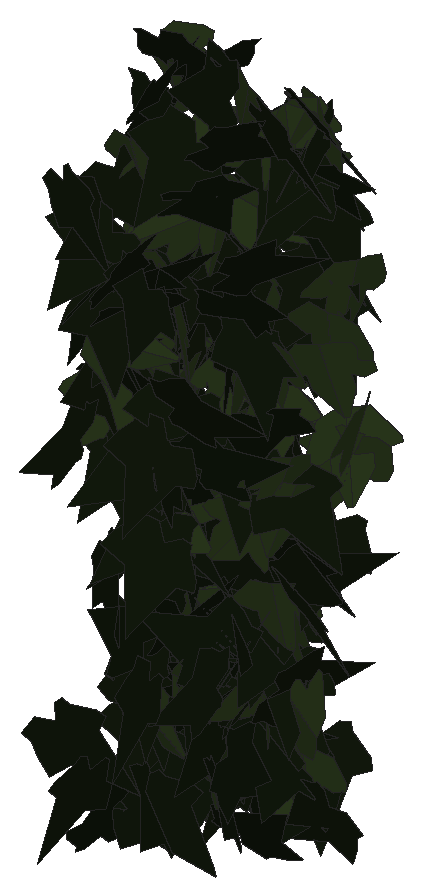
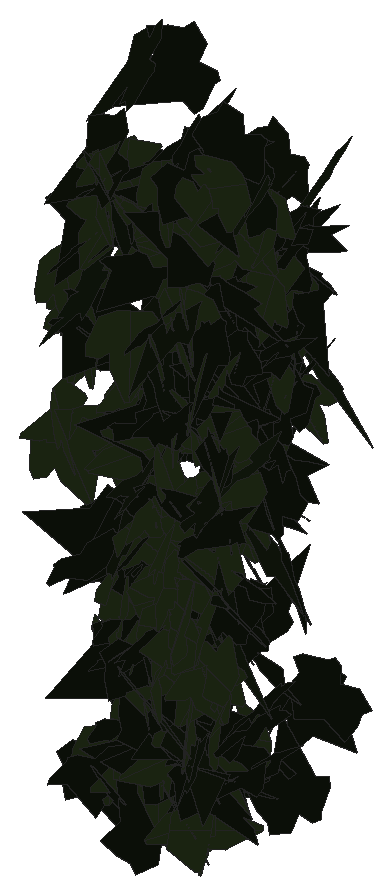
# SketchUp Ruby script. Lengths in inches.
U = 1.inch
M = Sketchup.active_model
def pt(a) = Geom::Point3d.new(a.map { |v| v * U })
def face(e, loops, mat)
  f = e.add_face(loops[0].map { |a| pt(a) })
  loops[1..].each { |l| e.add_face(l.map { |a| pt(a) }).erase! }
  f.material = f.back_material = mat if mat
  f
end
# faces: each face lists its corners as indices into pts; further lists are holes
def faces(e, pts, list, mat = nil) = list.each { |f| face(e, (f[0].is_a?(Array) ? f : [f]).map { |l| l.map { |i| pts[i] } }, mat) }
# xy, xz, yz: faces in a plane at the given z, y or x. An outline is a flat list of corners, or four numbers for a rectangle; further outlines are holes
def ring(l) = l.size == 4 ? [[l[0], l[1]], [l[2], l[1]], [l[2], l[3]], [l[0], l[3]]] : l.each_slice(2).to_a
def flat(e, list, mat, &to3) = list.each { |f| face(e, (f[0].is_a?(Array) ? f : [f]).map { |l| ring(l).map { |u, v| to3.(u, v) } }, mat) }
def xy(e, z, list, mat = nil) = flat(e, list, mat) { |x, y| [x, y, z] }
def xz(e, y, list, mat = nil) = flat(e, list, mat) { |x, z| [x, y, z] }
def yz(e, x, list, mat = nil) = flat(e, list, mat) { |y, z| [x, y, z] }
def lines(e, pts, list) = list.each { |a, b| e.add_line(pt(pts[a]), pt(pts[b])) }
# prism: a flat outline (further loops are holes) pulled along v
def prism(e, loops, v, mat = nil)
  f = face(e, loops, mat); d = Geom::Vector3d.new(v.map { |x| x * U })
  f.pushpull(f.normal.samedirection?(d) ? d.length : -d.length)
end
def box(e, o, s, mat = nil) = prism(e, [[o, [o[0] + s[0], o[1], o[2]], [o[0] + s[0], o[1] + s[1], o[2]], [o[0], o[1] + s[1], o[2]]]], [0, 0, s[2]], mat)
def at(x, y, z, deg = 0) = Geom::Transformation.translation(pt([x, y, z])) * Geom::Transformation.rotation(ORIGIN, Z_AXIS, deg.degrees)
def axes(o, x, y, z) = Geom::Transformation.new([*x, 0, *y, 0, *z, 0, *pt(o).to_a, 1])
def part(name) = M.definitions.add(name)
# library, detail: a bought-in or finely detailed component or shape, given as its bounding box
def library(name, o, s) = part(name).tap { |d| box(d.entities, o, s) }
def detail(e, o, s) = box(e.add_group.entities, o, s)
def put(e, d, t, mat = nil) = e.add_instance(d, t).tap { |i| i.material = mat if mat }
def group(e, t, mat = nil) = e.add_group.tap { |g| g.transformation = t; g.material = mat if mat }.entities
root = M.entities
M.materials.add("efeu1").color = [18, 25, 13]
M.materials.add("efeu2").color = [43, 57, 29]
c1 = part("ivyleaf_9")
p = [[1.54,2.16,1.25],[1.36,2.04,1.19],[-0.21,0.99,0.68],[-0.71,1.11,0.82],[-0.85,0.86,0.67],[-0.8,0.17,0.21],
  [-0.9,-0.01,0.1],[-0.67,-0.16,-0.02],[-0.08,-0.08,-0.05],[-0.03,-0.6,-0.4],[0.65,-0.88,-0.66],[0.83,-0.6,-0.49],
  [1.29,-0.42,-0.43],[1.8125,-0.07,-0.26],[1.21,0.44,0.15]]
faces(c1.entities,p,[[0,1,2,3,4,5,6,7,8,9,10,11,12,13,14]],"efeu1")
c2 = part("ivyleaf_10")
p = [[0,0.5,-0.03],[-0.0625,2.02,-0.43],[-0.19,2.01,-0.46],[-0.54,1.05,-0.29],[-0.52,0.625,-0.18],[-0.83,0.76,-0.28],
  [-1.16,0.64,-0.33],[-1.15,0.33,-0.24],[-0.77,-0.39,0.02],[-0.3,-0.51,0.16],[0.04,-0.48,0.23],[-0.02,2.01,-0.4375],
  [-0.06,2.01,-0.43],[0.04,-0.49,0.23],[0.67,-0.49,0.14],[1.38,0.36,-0.2],[1.375,0.51,-0.24],[0.81,0.65,-0.19],
  [0.62,0.59,-0.15],[0.6,1.09,-0.28],[0.5,1.23,-0.31]]
faces(c2.entities,p,[[0,1,2,3,4,5,6,7,8,9,10],[11,12,0,13,14,15,16,17,18,19,20]],"efeu2")
put(root,c1,axes([7.01,222.2,232.59],[-0.0861,0.39722,-0.16472],[-0.12182,0.13587,0.41345],[0.44549,0.11392,0.08122]))
put(root,c1,axes([6.7,222.25,227.66],[0.03553,-0.01472,0.45084],[0.36359,-0.27327,-0.03622],[0.29539,0.33813,-0.00964]))
put(root,c1,axes([7.11,222.03,228.04],[-0.32073,-0.31158,0.06535],[-0.03827,-0.05301,-0.44751],[0.34115,-0.29888,0.01124]))
put(root,c1,axes([6.91,222.69,224.36],[0.0032,-0.43244,-0.04889],[-0.00048,0.04701,-0.44975],[0.46979,0.00299,-0.00012]))
put(root,c1,axes([7.0625,223.45,227.76],[-0.18053,-0.37603,0.14665],[-0.05909,-0.12998,-0.42796],[0.42968,-0.17587,0.00276]))
put(root,c1,axes([6.99,222.54,223.62],[-0.14612,-0.39297,0.13356],[0.0204,-0.14086,-0.42757],[0.44603,-0.12229,0.06331]))
put(root,c1,axes([6.82,222.83,232.54],[0.18169,-0.38646,0.11189],[0.06107,-0.09265,-0.43809],[0.42892,0.17689,0.01498]))
put(root,c2,axes([7.1,223.21,226.51],[-0.18859,0.36961,0.15468],[-0.06703,0.13518,-0.42513],[-0.42504,-0.18531,-0.00159]))
put(root,c1,axes([7.1,222.16,229.875],[-0.22078,-0.35941,0.14054],[-0.05471,-0.12651,-0.42963],[0.41107,-0.20987,0.0183]))
put(root,c1,axes([7.45,222.82,229.3125],[-0.12494,0.12692,0.41565],[-0.38106,0.19459,-0.17048],[-0.24474,-0.36776,0.05325]))
put(root,c1,axes([6.84,221.78,226.36],[-0.08829,-0.08514,-0.43543],[0.46005,-0.04918,-0.0761],[-0.03566,-0.42374,0.09632]))
put(root,c1,axes([6.8125,220.86,224.3],[-0.02656,-0.02098,-0.45115],[0.31827,0.31835,-0.03339],[0.34454,-0.2957,-0.00394]))
put(root,c1,axes([7.1,221.54,231.39],[-0.08179,-0.2223,0.38081],[-0.13532,-0.34408,-0.2442],[0.44239,-0.14635,-0.00429]))
put(root,c2,axes([7.2,223.46,232.61],[-0.20216,-0.2018,-0.35032],[-0.15461,-0.31241,0.27738],[-0.39489,0.22562,0.07074]))
put(root,c1,axes([7.33,221.87,226.84],[-0.3534,0.27782,-0.0733],[0.05803,-0.04561,-0.44642],[-0.30406,-0.3316,-0.00001]))
put(root,c2,axes([6.8,223.39,225.49],[-0.17295,-0.02757,0.41965],[0.43654,0.00431,0.16714],[-0.01532,0.4341,0.02499]))
put(root,c1,axes([6.98,222.47,224.53],[0.01298,-0.42928,0.07202],[-0.01082,-0.06953,-0.44646],[0.4695,0.01027,-0.01228]))
put(root,c1,axes([7.07,222.28,228.86],[-0.10618,0.02563,0.43989],[-0.04943,-0.43231,0.01618],[0.45497,-0.04099,0.10442]))
put(root,c2,axes([7.16,222,232.21],[-0.46772,0.03923,-0.01202],[0.01235,-0.00189,-0.45224],[-0.0424,-0.43322,0.00088]))
put(root,c2,axes([7.26,221.2,229.75],[-0.26529,0.29838,0.20763],[-0.18922,0.11151,-0.39751],[-0.33842,-0.29625,0.05949]))
put(root,c2,axes([7.2,221.3,229.04],[0.43956,0.01533,-0.1589],[-0.16486,-0.00662,-0.42358],[-0.01801,0.43468,-0.00085]))
put(root,c2,axes([7.4,222.88,228.48],[-0.03279,0.12694,0.43155],[-0.38872,0.22499,-0.09897],[-0.26179,-0.34998,0.09291]))
put(root,c1,axes([7.27,221.23,230.55],[-0.10332,0.35928,-0.23484],[0.07647,-0.21472,-0.38649],[-0.45187,-0.11849,-0.01171]))
put(root,c1,axes([7.02,221.47,222.54],[0.25576,0.28595,0.23572],[-0.15701,-0.17389,0.38613],[0.36145,-0.27788,0.00093]))
put(root,c2,axes([7.18,221.93,230.82],[-0.44666,0.13446,-0.01027],[0.01193,0.00205,-0.45225],[-0.14512,-0.41369,-0.00558]))
put(root,c1,axes([7.01,221.79,231.97],[0.06022,-0.27008,-0.34987],[-0.02363,0.337,-0.28515],[0.46533,0.05206,0.03079]))
put(root,c2,axes([7.16,223.29,225.375],[0.30448,0.30754,-0.12804],[-0.09164,-0.08924,-0.4339],[-0.34584,0.29441,0.00224]))
put(root,c1,axes([7,221.58,229.33],[0.33209,0.24469,0.19401],[0.15576,0.11835,-0.40868],[-0.29354,0.33962,0.00263]))
put(root,c1,axes([7.48,221.77,224.82],[-0.41542,0.05328,-0.20389],[-0.20887,0.03249,0.40382],[0.06718,0.4305,-0.00524]))
put(root,c2,axes([7.45,223.32,222.92],[0.03944,0.06073,-0.49473],[-0.41349,-0.27314,-0.06649],[-0.27834,0.41437,0.02868]))
put(root,c2,axes([6.875,223.14,233.12],[-0.19368,0.00219,-0.41216],[0.42798,-0.00512,-0.18652],[-0.00601,-0.43496,0.00012]))
put(root,c1,axes([6.93,222.91,228.41],[0.0057,-0.43914,0.239],[0.18695,-0.21981,-0.40833],[0.4637,0.09402,0.16169]))
put(root,c1,axes([7.24,223.38,227.88],[0.217,-0.37827,0.079],[-0.03153,0.07049,0.44539],[-0.41549,-0.20291,0.00746]))
put(root,c1,axes([7.12,221.57,229.04],[0.19452,-0.28428,-0.28665],[0.15821,-0.23348,0.34999],[-0.39729,-0.23217,-0.00097]))
put(root,c1,axes([7.45,222.55,225.64],[-0.3255,0.31364,0.00457],[-0.0036,0.0029,-0.45238],[-0.33874,-0.30141,0.00041]))
put(root,c1,axes([7.26,221.32,231.35],[-0.30896,-0.30466,0.12552],[-0.03057,-0.13664,-0.42849],[0.35259,-0.27881,0.07284]))
put(root,c2,axes([7.27,222.34,231.84],[0.21821,0.30996,-0.23791],[-0.15757,-0.1775,-0.38414],[-0.38506,0.24828,0.02238]))
put(root,c2,axes([7.3,223.26,230.14],[-0.28074,0.30803,0.17017],[-0.12216,0.11859,-0.41907],[-0.35633,-0.28334,0.00959]))
put(root,c1,axes([7.5,220.38,228.87],[-0.34524,0.28997,0.05653],[-0.04568,0.03427,-0.44884],[-0.31533,-0.32244,0.00313]))
put(root,c1,axes([7.35,222.44,226.51],[0.01971,0.17276,0.41476],[0.01942,0.39851,-0.1804],[-0.46898,0.02376,0.00996]))
put(root,c1,axes([7.12,222.58,233.54],[0.44489,0.11923,-0.07587],[-0.07445,-0.02421,-0.44597],[-0.13132,0.41764,-0.0042]))
put(root,c1,axes([7.04,220.71,232.24],[0.28743,-0.33046,-0.09969],[-0.06297,0.07612,-0.44127],[0.36624,0.27244,0.00237]))
put(root,c1,axes([6.85,221.91,228.97],[0.2343,-0.16249,0.35384],[0.3202,-0.16898,-0.28055],[0.25157,0.36642,0.02753]))
put(root,c2,axes([7.2,222.625,229.98],[-0.09056,0.42418,-0.0495],[0.00675,-0.04728,-0.44967],[-0.46094,-0.08403,0.00314]))
put(root,c1,axes([7.125,222.78,228.55],[0.1144,0.34859,0.24718],[-0.09401,-0.22172,0.37855],[0.44586,-0.13619,0.0164]))
put(root,c1,axes([7.55,223.03,226.71],[-0.43011,0.15738,0.07959],[-0.07961,0.02168,-0.44529],[-0.17141,-0.40495,0.0071]))
put(root,c1,axes([7.43,223,223.74],[-0.10007,0.30049,-0.3126],[0.01008,-0.30612,-0.32127],[-0.45891,-0.07225,0.06111]))
put(root,c1,axes([6.96,222.11,228.7],[-0.04751,-0.03905,-0.44824],[0.46005,0.07258,-0.05205],[0.08252,-0.42712,0.03213]))
put(root,c1,axes([7.11,222.59,223.98],[0.40028,0.22007,0.06087],[0.06004,0.02099,-0.44816],[-0.23849,0.37464,-0.01065]))
put(root,c2,axes([7,222.7,228.3],[-0.18205,-0.05521,-0.41308],[0.41661,0.09541,-0.18405],[0.11835,-0.4208,0.01247]))
put(root,c1,axes([7.32,223.03,230.66],[0.36273,0.00889,-0.28735],[-0.29807,-0.01401,-0.34938],[-0.01702,0.43468,-0.00538]))
put(root,c1,axes([7.48,223.31,233.16],[-0.11581,0.33752,-0.2627],[-0.01717,-0.26369,-0.35943],[-0.45498,-0.07596,0.08043]))
put(root,c1,axes([7.09,221.73,230.03],[0.13846,0.411,-0.06466],[0.00846,0.06266,0.44761],[0.44885,-0.12797,0.01151]))
put(root,c1,axes([7.38,222.66,230.24],[0.30947,0.20995,-0.26112],[-0.24035,-0.1197,-0.36824],[-0.25918,0.36169,0.0297]))
put(root,c1,axes([7.07,222.88,229.81],[-0.17981,-0.09387,-0.40639],[0.39385,0.14245,-0.19718],[0.18238,-0.40015,0.02514]))
put(root,c1,axes([7.26,222.05,228.01],[-0.29092,0.09172,-0.34218],[0.33517,-0.10928,-0.29593],[-0.15406,-0.41094,0.00233]))
put(root,c1,axes([7.53,222.6,231.04],[-0.46728,-0.02463,0.03915],[-0.04018,-0.00864,-0.45065],[0.02731,-0.43422,0.00674]))
put(root,c2,axes([7,222.85,229.13],[0.21355,0.11427,0.38504],[0.3392,0.19614,-0.23741],[-0.24505,0.37108,0.00691]))
put(root,c2,axes([7.48,222.95,223.62],[0.35413,0.09351,-0.28093],[-0.28817,-0.04734,-0.35389],[-0.11075,0.42219,0.02254]))
put(root,c1,axes([7.2,222.88,225.96],[0.45213,-0.05395,0.10934],[-0.11209,0.01716,0.43897],[-0.06101,-0.4313,0.00379]))
put(root,c2,axes([7.04,222.31,224.01],[-0.14654,0.09861,-0.41742],[0.36626,-0.21489,-0.17414],[-0.25513,-0.36514,-0.01025]))
put(root,c2,axes([7.41,221.57,228.47],[-0.2646,0.34109,0.11792],[-0.10009,0.07264,-0.43551],[-0.37507,-0.26001,0.03302]))
put(root,c1,axes([7.14,222.19,229.67],[0.14557,-0.46305,-0.11997],[-0.01192,0.12185,-0.48478],[0.47819,0.144,0.02444]))
put(root,c2,axes([7.16,223.05,224.37],[-0.0448,-0.13855,0.47833],[0.31805,-0.37751,-0.07956],[0.3832,0.29713,0.12196]))
put(root,c1,axes([7.53,222.86,224.05],[0.02416,0.42314,0.1023],[-0.06245,0.10052,-0.43603],[-0.465,0.00848,0.06388]))
put(root,c2,axes([7.42,221.51,230.85],[-0.27853,-0.34877,-0.03408],[0.021,0.02637,-0.45111],[0.37774,-0.25863,-0.00005]))
put(root,c1,axes([7.44,222.6,226.54],[-0.4272,-0.14138,-0.11752],[0.11884,0.02777,-0.43673],[0.1552,-0.41044,0.01093]))
put(root,c1,axes([7.42,220.69,223.86],[-0.08673,0.19549,-0.39542],[0.17744,-0.34304,-0.21952],[-0.42627,-0.18257,-0.01093]))
put(root,c1,axes([7.19,222.29,229.53],[0.04562,0.04522,0.4478],[0.38757,0.23836,-0.06265],[-0.26157,0.36106,-0.01473]))
put(root,c2,axes([7.35,222.99,225.29],[-0.39543,-0.16822,-0.17047],[0.15913,0.0719,-0.41904],[0.19754,-0.39466,-0.00368]))
put(root,c2,axes([7.52,222.87,222.99],[-0.37289,0.23265,0.13109],[-0.12784,0.04952,-0.43227],[-0.25558,-0.36421,0.02496]))
put(root,c2,axes([7.22,221.82,229.58],[-0.35666,-0.00544,-0.29441],[0.30555,-0.02324,-0.34279],[-0.01188,-0.43434,0.02203]))
put(root,c1,axes([7.69,223.04,223.6],[-0.44283,-0.01562,0.15019],[-0.14282,-0.13881,-0.40609],[0.06491,-0.41196,0.13113]))
put(root,c2,axes([7.69,223.15,229.09],[0.1827,0.15413,0.38473],[-0.35458,-0.17696,0.23282],[0.2482,-0.36627,0.04942]))
put(root,c1,axes([7.48,221.6875,225.38],[0.05055,0.05794,0.44572],[-0.28565,-0.33723,0.07745],[0.36954,-0.2686,-0.0011]))
put(root,c2,axes([7.53,223.16,224.64],[0.13665,-0.23106,-0.36001],[-0.08108,0.3432,-0.26679],[0.44211,0.13436,0.06234]))
put(root,c2,axes([7.53,223.43,225.88],[-0.28222,0.34622,-0.03397],[-0.02308,0.02479,0.45112],[0.37487,0.26218,0.00221]))
put(root,c2,axes([7.29,222.88,226.66],[-0.17893,-0.22953,0.3435],[0.25269,0.23556,0.2923],[-0.35333,0.2847,0.03509]))
put(root,c2,axes([7.55,222.85,228.96],[0.06217,-0.42943,0.04027],[0.00081,-0.03896,-0.45058],[0.46567,0.0574,-0.0046]))
put(root,c1,axes([7.71,221.73,228.12],[-0.35214,-0.19953,0.21591],[-0.18597,-0.11625,-0.39746],[0.24925,-0.36864,0.00848]))
put(root,c1,axes([7.9,221.88,227.7],[-0.34525,0.20754,0.21805],[-0.25468,0.00601,-0.38011],[-0.19145,-0.38225,0.11241]))
put(root,c1,axes([7.38,223.46,223.68],[-0.03749,-0.1454,0.42485],[0.04586,-0.40898,-0.14764],[0.46605,0.02855,0.0487]))
put(root,c1,axes([7.68,222.59,223.09],[-0.2437,-0.18582,0.33503],[-0.20472,-0.26671,-0.29809],[0.34556,-0.28907,0.05967]))
put(root,c2,axes([7.4375,221.86,228.46],[0.30978,0.30431,0.12456],[0.07891,0.09565,-0.43474],[-0.34427,0.29575,0.01244]))
put(root,c2,axes([7.31,223.05,222.98],[0.12103,0.1092,0.42212],[0.27625,0.3156,-0.16176],[-0.36021,0.27874,0.01778]))
put(root,c2,axes([7.55,222.93,225.1875],[-0.42514,0.17088,-0.07404],[0.06958,-0.03038,-0.44629],[-0.18743,-0.39888,0.00227]))
put(root,c1,axes([7.35,222.59,224.44],[0.46069,0.05988,0.06309],[0.06192,0.02755,-0.44754],[-0.06813,0.42998,0.01989]))
put(root,c1,axes([7.55,221.22,231],[0.37486,0.24134,-0.10661],[-0.09487,-0.05322,-0.43961],[-0.26682,0.35798,0.00652]))
put(root,c2,axes([7.31,221.18,229.91],[-0.08431,-0.09004,-0.43509],[0.43691,0.12314,-0.10607],[0.1507,-0.40738,0.06411]))
put(root,c2,axes([7.73,223.2,227.68],[-0.04563,0.0674,0.44477],[-0.07365,-0.42537,0.06272],[0.46174,-0.06119,0.05396]))
put(root,c1,axes([7.37,222.42,226.07],[0.42961,-0.17597,-0.0054],[-0.00416,0.00411,-0.45236],[0.19008,0.3978,0.00229]))
put(root,c2,axes([7.59,223.625,226.79],[-0.04936,0.22659,-0.38324],[-0.01642,-0.37116,-0.2354],[-0.46691,-0.0109,0.04879]))
put(root,c1,axes([7.51,223.5,229.45],[-0.08394,-0.40195,-0.15291],[0.03979,0.1426,-0.42568],[0.46052,-0.08558,0.0089]))
put(root,c2,axes([7.77,222.26,231.33],[-0.08924,-0.03821,0.44238],[-0.10528,-0.42013,-0.05895],[0.44907,-0.10609,0.07409]))
put(root,c1,axes([7.73,222.43,226.48],[0.12819,-0.07586,-0.42802],[-0.36743,0.23163,-0.14644],[0.2632,0.3603,0.00403]))
put(root,c1,axes([7.4375,222.51,227.375],[-0.11027,-0.00567,-0.43972],[0.44334,-0.10568,-0.10162],[-0.10956,-0.42193,0.03136]))
put(root,c2,axes([7.72,223.1,231.03],[0.22306,-0.35675,-0.14447],[-0.06138,0.12752,-0.42847],[0.40889,0.21376,0.01449]))
put(root,c2,axes([7.61,221.81,228.12],[-0.41036,-0.14536,-0.16018],[0.15309,0.0605,-0.42305],[0.16994,-0.40551,-0.0057]))
put(root,c1,axes([7.42,222.24,226.99],[0.30975,-0.31728,-0.08256],[0.01771,0.1194,-0.43469],[0.35278,0.27259,0.09431]))
put(root,c1,axes([7.84,221.77,227.31],[-0.41673,-0.18555,0.07993],[-0.06046,-0.0605,-0.4442],[0.20831,-0.38876,0.03098]))
put(root,c2,axes([7.9375,223.42,225.9],[-0.0736,-0.03331,0.44547],[-0.27471,-0.34638,-0.0701],[0.37394,-0.26103,0.03618]))
put(root,c2,axes([7.83,221.65,227.92],[0.16419,-0.15422,-0.39236],[-0.16012,0.35414,-0.21269],[0.41002,0.20006,0.07405]))
put(root,c1,axes([7.625,222.76,230.93],[-0.13014,-0.41732,-0.02431],[0.00718,0.02241,-0.45175],[0.45136,-0.12068,0.00018]))
put(root,c1,axes([7.33,222.02,225.57],[0.37195,-0.07462,0.26524],[0.27147,-0.04395,-0.36638],[0.0931,0.42629,0.00865]))
put(root,c2,axes([7.57,222.1,227.18],[0.40704,0.15575,0.15746],[0.11987,0.12254,-0.41845],[-0.20165,0.38724,0.06909]))
put(root,c1,axes([7.58,221.9,222.97],[0.00769,-0.24832,0.37137],[0.01559,-0.35681,-0.25834],[0.46948,0.01591,0.00249]))
put(root,c1,axes([7.6,222.86,231.81],[0.06507,0.3992,-0.16845],[-0.0372,0.16749,0.41598],[0.46378,-0.04257,0.057]))
put(root,c1,axes([7.6,220.97,230.71],[-0.25187,-0.26824,-0.2608],[0.30016,0.06521,-0.34135],[0.25919,-0.33619,0.14187]))
put(root,c2,axes([7.74,221.84,227.11],[0.34775,0.27359,-0.10757],[-0.08475,-0.06739,-0.43942],[-0.3043,0.33141,-0.00055]))
put(root,c2,axes([7.42,223.39,225.93],[-0.00363,0.00976,-0.45227],[0.42276,-0.18958,-0.00757],[-0.20486,-0.39139,-0.00761]))
put(root,c2,axes([7.78,223.42,228.62],[0.10229,-0.41167,0.108],[0.03896,-0.09821,-0.43912],[0.45687,0.10054,0.01327]))
put(root,c2,axes([7.5,222.91,232.07],[-0.05154,-0.07935,-0.44203],[0.40344,0.20776,-0.08396],[0.23514,-0.37385,0.04717]))
put(root,c2,axes([7.65,223.3,226.59],[0.40404,0.20503,0.08842],[0.0752,0.0498,-0.44355],[-0.22761,0.38041,0.01041]))
put(root,c1,axes([7.91,223.23,229.9],[-0.2813,0.27138,-0.22722],[0.15662,-0.16359,-0.39112],[-0.34212,-0.29802,0.00778]))
put(root,c1,axes([7.84,220.99,230.625],[0.16831,0.40497,-0.03187],[-0.01603,-0.02712,-0.45126],[-0.43832,0.15649,0.00427]))
put(root,c1,axes([7.99,223.64,228.04],[-0.4231,-0.15275,0.11587],[-0.10445,-0.05836,-0.43688],[0.17546,-0.40309,0.01935]))
put(root,c2,axes([7.64,223.1,231.07],[0.44251,0.09752,0.11315],[0.11309,0.02989,-0.43799],[-0.11004,0.42287,0.00487]))
put(root,c1,axes([7.61,222.17,225.18],[0.15412,0.41013,0.02666],[-0.03219,-0.01673,0.451],[0.44263,-0.14402,0.02352]))
put(root,c2,axes([7.88,223.08,230.72],[-0.05561,-0.08276,-0.4409],[-0.16159,-0.39709,0.09952],[-0.43762,0.15714,0.01928]))
put(root,c2,axes([7.73,223.1875,230.43],[0.33345,-0.28616,0.11398],[0.09336,-0.06792,-0.43771],[0.3175,0.32051,0.00901]))
put(root,c2,axes([7.67,221.65,228.44],[-0.00714,-0.34229,0.27909],[0.23873,-0.23379,-0.30446],[0.40456,0.13192,0.18459]))
put(root,c1,axes([7.61,221.66,223.1875],[-0.07626,-0.13366,-0.42421],[0.21021,0.35846,-0.1572],[0.41317,-0.20704,0.00169]))
put(root,c2,axes([7.8,223.34,227.37],[-0.17784,0.40062,-0.04183],[0.0172,-0.03693,-0.45046],[-0.4345,-0.16543,-0.00072]))
put(root,c2,axes([8.06,223.17,232.83],[-0.39004,0.09808,0.23063],[-0.23083,0.05914,-0.38919],[-0.12369,-0.41965,-0.00094]))
put(root,c1,axes([7.79,223.02,230.89],[0.43919,0.00036,-0.23899],[-0.23177,0.12265,-0.42572],[0.05832,0.48472,0.1079]))
put(root,c2,axes([7.91,223.13,224.68],[0.27367,0.41711,0.03352],[-0.03416,-0.01764,0.49852],[0.41706,-0.27515,0.01884]))
put(root,c1,axes([7.99,223.29,224.13],[0.24903,0.09175,0.37156],[-0.38698,-0.04434,0.25234],[0.0946,-0.4229,0.05415]))
put(root,c2,axes([7.86,223.57,227.95],[0.07517,0.35716,-0.2479],[-0.04826,-0.23415,-0.37843],[-0.46123,0.08271,-0.00081]))
put(root,c1,axes([7.625,221.26,230.65],[0.21406,0.36434,-0.13639],[0.0727,0.11266,0.43132],[0.41183,-0.20926,-0.00525]))
put(root,c1,axes([7.74,222.7,223.91],[0.2048,-0.34241,-0.19737],[-0.09782,0.16678,-0.40707],[0.41134,0.21015,0.00147]))
put(root,c1,axes([8.01,223.1,223.15],[-0.4162,0.09562,-0.1848],[0.18689,-0.04042,-0.41293],[-0.11209,-0.42243,-0.00232]))
put(root,c2,axes([8.08,222.79,228.875],[0.05512,0.03045,-0.44816],[-0.16471,0.40725,0.01114],[0.43652,0.14982,0.06079]))
put(root,c2,axes([7.78,222.07,230],[-0.18926,0.27616,-0.29826],[0.15745,-0.24707,-0.34008],[-0.40013,-0.22785,0.00726]))
put(root,c1,axes([7.83,221.64,227.93],[0.37175,0.2618,0.04884],[0.03603,0.03371,-0.4497],[-0.28499,0.34576,0.00686]))
put(root,c2,axes([7.99,222.34,225.07],[0.06175,-0.40298,0.15965],[0.01,-0.15367,-0.42312],[0.46562,0.05674,-0.01209]))
put(root,c2,axes([8.18,223.23,226.15],[0.10938,0.13675,0.41635],[-0.24538,-0.32966,0.17688],[0.38541,-0.24869,-0.00554]))
put(root,c1,axes([7.9,222.55,224.04],[0.19763,0.21464,0.34441],[0.15341,0.30475,-0.28704],[-0.39764,0.22424,0.06043]))
put(root,c2,axes([8.02,222.89,228.93],[0.26579,0.29432,-0.21322],[-0.1522,-0.1493,-0.39884],[-0.35623,0.28339,0.01132]))
put(root,c2,axes([8.18,223.23,225.05],[0.15868,-0.06012,-0.4212],[-0.23276,0.35449,-0.13604],[0.37598,0.24483,0.09354]))
put(root,c2,axes([8.03,223.33,230.26],[0.26655,-0.34776,-0.08931],[-0.04097,0.07832,-0.44325],[0.38469,0.2493,0.01468]))
put(root,c1,axes([8.04,222.71,232.96],[-0.10711,-0.0348,0.439],[-0.1837,-0.39376,-0.07532],[0.41892,-0.18157,0.07921]))
put(root,c1,axes([8.13,223.52,229.09],[-0.39867,-0.29357,0.06983],[-0.0618,-0.03382,-0.49501],[0.29537,-0.40332,-0.00932]))
put(root,c2,axes([8.12,222.88,228.23],[-0.18967,0.27808,0.29608],[-0.18693,0.22684,-0.34148],[-0.38703,-0.24584,0.01982]))
put(root,c2,axes([7.87,223.04,223.79],[-0.05436,-0.06178,-0.44474],[0.25144,0.35881,-0.08241],[0.39311,-0.23804,-0.00879]))
put(root,c2,axes([7.9375,222.72,231.55],[-0.00231,-0.44476,0.22843],[0.18008,-0.21384,-0.41454],[0.46644,0.08036,0.16118]))
put(root,c1,axes([8.26,222.87,224.42],[-0.33219,0.30717,-0.01699],[0.01248,-0.01154,-0.45208],[-0.33198,-0.3078,0]))
put(root,c2,axes([8.23,223.4,227.27],[0.29073,0.1209,-0.33238],[-0.33804,-0.07597,-0.30407],[-0.14804,0.4109,0.04157]))
put(root,c1,axes([8.09,221.29,228.34],[0.25189,-0.09264,-0.36953],[-0.33051,0.18358,-0.25869],[0.21916,0.38333,0.03459]))
put(root,c2,axes([8.2,223.12,223.75],[-0.46137,-0.17719,0.07578],[-0.07215,-0.0235,-0.49421],[0.1787,-0.46696,-0.00388]))
put(root,c2,axes([7.94,222.82,223.8],[-0.35237,0.13041,-0.26671],[0.18916,-0.21758,-0.34681],[-0.24651,-0.35338,0.11512]))
put(root,c1,axes([8.44,223.24,224.79],[-0.28815,0.32796,0.24375],[-0.18818,0.15825,-0.43537],[-0.36271,-0.34264,0.03223]))
put(root,c1,axes([8.07,222.82,229.02],[0.40327,0.12375,-0.19312],[-0.19288,-0.05129,-0.40905],[-0.14449,0.41386,0.00706]))
put(root,c1,axes([7.75,223.26,229.58],[0.11489,-0.21319,0.37851],[0.27527,-0.26657,-0.23988],[0.36296,0.26966,0.06211]))
put(root,c1,axes([8.16,221.88,232.7],[-0.33115,-0.30094,0.07087],[-0.03022,-0.06855,-0.4458],[0.33187,-0.30653,0.03012]))
put(root,c1,axes([7.98,222.57,223.89],[0.05518,-0.11862,-0.432],[0.30499,-0.30736,0.12741],[-0.35305,-0.28405,0.04254]))
put(root,c1,axes([8.04,222.625,224.72],[0.41686,0.18094,-0.09007],[-0.08755,-0.0311,-0.4433],[-0.19817,0.39436,0.00637]))
put(root,c1,axes([7.99,223.3,230.65],[-0.00887,-0.43293,0.04322],[-0.00295,-0.04151,-0.45033],[0.46971,-0.00844,-0.00201]))
put(root,c1,axes([7.95,223.39,225.82],[0.15107,-0.35024,-0.22544],[-0.03903,0.21761,-0.38992],[0.44313,0.13857,0.04252]))
put(root,c1,axes([8.39,222.24,225.24],[-0.01493,0.01046,0.45204],[-0.45197,-0.11825,-0.01088],[0.12733,-0.41849,0.01438]))
put(root,c1,axes([7.9375,222.42,229.87],[-0.20925,-0.04506,0.40233],[0.38946,-0.18397,0.16554],[0.15889,0.3916,0.12407]))
put(root,c2,axes([8.25,222.35,223.36],[0.05712,0.01069,0.44891],[-0.21345,0.38723,0.01521],[-0.4146,-0.19789,0.05401]))
put(root,c1,axes([8.34,223.29,225.38],[-0.03857,0.31653,-0.30809],[-0.02963,-0.2983,-0.32803],[-0.46728,-0.00721,0.04623]))
put(root,c1,axes([7.98,223.31,222.52],[0.32127,0.30829,0.07848],[-0.05969,-0.05152,0.44552],[0.33755,-0.30253,0.00409]))
put(root,c1,axes([8.03,223.72,228.2],[0.02644,-0.33719,0.28468],[0.03247,-0.27219,-0.3515],[0.46793,0.03794,0.0083]))
put(root,c1,axes([7.96,223.5625,228.45],[0.26966,-0.35262,0.0524],[0.036,-0.03813,-0.44932],[0.38301,0.25185,0.00534]))
put(root,c1,axes([8.35,222.86,226.12],[0.30861,0.00693,0.39334],[-0.39213,0.04558,0.30685],[-0.0316,-0.49787,0.03357]))
put(root,c1,axes([7.875,223.06,223.64],[0.25377,-0.00031,0.38072],[0.39532,0.00679,-0.24434],[-0.006,0.43495,0.00408]))
put(root,c1,axes([8.37,223.27,225.24],[-0.40454,-0.28981,0.04857],[-0.0376,-0.03091,-0.49763],[0.29143,-0.40627,0.00321]))
put(root,c1,axes([8.29,221.15,228.75],[-0.40531,-0.18794,-0.11887],[0.12412,0.02519,-0.43554],[0.20255,-0.3915,0.02904]))
put(root,c1,axes([8.39,222.86,225.3],[-0.28954,0.25679,-0.23581],[0.15287,-0.17916,-0.38507],[-0.33691,-0.30197,0.02794]))
put(root,c1,axes([8.27,221.65,229.12],[-0.27785,-0.34819,-0.04411],[0.03084,0.03164,-0.45022],[0.37757,-0.25882,0.00431]))
put(root,c2,axes([8.43,222.9,223.99],[0.30477,-0.24328,-0.31293],[-0.16881,0.27749,-0.38013],[0.35863,0.33736,0.08701]))
put(root,c1,axes([8.37,219.99,231.68],[0.07898,0.34972,0.25806],[0.05832,0.24221,-0.37157],[-0.45943,0.09087,-0.0028]))
put(root,c1,axes([8.3,221.08,227.31],[-0.19438,-0.39028,0.06984],[-0.01984,-0.06546,-0.44684],[0.42724,-0.18061,0.01102]))
put(root,c1,axes([8.125,222.72,229.52],[-0.03223,-0.03569,-0.44981],[0.42115,-0.19246,-0.01146],[-0.20569,-0.38847,0.047]))
put(root,c1,axes([8.34,220.73,225.46],[-0.36666,0.03994,-0.27977],[0.28312,-0.06647,-0.35434],[-0.07818,-0.42803,0.02892]))
put(root,c1,axes([8,222.98,228.77],[0.26175,0.01371,0.3754],[0.37378,0.11567,-0.24625],[-0.11173,0.41911,0.05568]))
put(root,c1,axes([8.09,223.33,231.47],[-0.04543,-0.24535,-0.371],[0.22357,0.30339,-0.2424],[0.41069,-0.19231,0.09091]))
put(root,c1,axes([8.15,223.27,227.23],[0.13758,-0.41144,-0.0634],[-0.0205,0.05794,-0.44793],[0.44874,0.12879,-0.00103]))
put(root,c2,axes([8.49,223.34,230.38],[-0.43618,-0.24056,0.04329],[-0.03763,-0.02141,-0.49812],[0.24151,-0.4378,0.00058]))
put(root,c1,axes([8.2,222.89,225.42],[0.06119,-0.27753,0.41138],[0.07865,-0.40383,-0.28413],[0.48997,0.09948,-0.00577]))
put(root,c1,axes([8.3,220.78,231.13],[-0.03587,-0.36309,0.24673],[0.03972,-0.23944,-0.37576],[0.46674,-0.00753,0.05094]))
put(root,c1,axes([8.45,221.52,232.27],[0.26804,0.35717,-0.00762],[-0.00409,-0.00629,-0.45234],[-0.38581,0.24822,-0.00049]))
put(root,c2,axes([8.51,222.84,224.49],[-0.26419,-0.4166,-0.08154],[0.04534,0.0678,-0.4933],[0.42207,-0.26805,0.00195]))
put(root,c2,axes([8.22,223.37,228.58],[-0.24552,-0.09018,-0.37413],[0.39649,0.00512,-0.24262],[0.0568,-0.42552,0.07637]))
put(root,c2,axes([8.58,222.41,229.45],[0.11752,-0.34415,-0.34315],[-0.01029,0.3512,-0.35574],[0.48588,0.09067,0.07546]))
put(root,c1,axes([8.82,222.66,227.77],[-0.05692,0.22925,0.44069],[-0.17015,0.40774,-0.23409],[-0.4667,-0.17661,0.03159]))
put(root,c2,axes([8.28,222.84,231.47],[0.19398,0.08341,0.4028],[0.2988,0.27798,-0.1957],[-0.30627,0.32403,0.0642]))
put(root,c2,axes([8.73,222.22,227.3],[0.38271,-0.01068,-0.26216],[-0.26074,0.11188,-0.35789],[0.07914,0.42023,0.08862]))
put(root,c1,axes([8.53,223.18,225.72],[-0.24026,-0.4365,-0.04181],[0.03077,0.03078,-0.4981],[0.43741,-0.24192,0.01207]))
put(root,c2,axes([8.54,223.125,223.34],[0.27228,0.35159,-0.04711],[-0.03182,-0.03461,-0.44992],[-0.38153,0.2538,0.0039]))
put(root,c1,axes([8.41,223.5625,227.03],[0.0134,-0.21011,0.39592],[0.07005,-0.37569,-0.21785],[0.46435,0.06274,0.02144]))
put(root,c2,axes([8.35,223.27,224.77],[0.25333,-0.2175,0.37218],[0.34107,-0.16286,-0.32733],[0.26361,0.41973,0.06585]))
put(root,c1,axes([8.91,221.35,225.34],[-0.38923,0.23826,0.05272],[-0.04516,0.02867,-0.44932],[-0.25918,-0.36281,-0.00089]))
put(root,c1,axes([8.54,223.09,225.33],[-0.16051,-0.4152,0.2277],[0.04871,-0.25363,-0.42813],[0.47102,-0.11526,0.12187]))
put(root,c2,axes([8.68,222.68,227.75],[0.48555,0.03093,-0.11524],[-0.11561,0.00251,-0.48644],[-0.02951,0.49904,0.00959]))
put(root,c2,axes([8.82,223.125,226.03],[-0.37621,0.24812,0.21656],[-0.18028,0.11999,-0.45067],[-0.27561,-0.41718,-0.00082]))
put(root,c1,axes([8.91,222.41,227.91],[-0.29721,0.33609,-0.02417],[0.01918,-0.0155,-0.45174],[-0.36334,-0.27574,-0.00407]))
put(root,c1,axes([8.38,222.6,222.51],[0.45009,0.07574,-0.10299],[0.10481,0.01982,0.44052],[0.08452,-0.4279,0.00218]))
put(root,c1,axes([8.62,221.98,230.59],[0.42229,0.18196,-0.05909],[-0.05436,-0.02651,-0.44851],[-0.19857,0.39423,-0.00289]))
put(root,c2,axes([8.67,223.11,225.58],[-0.37437,0.29747,-0.14614],[0.10046,-0.10824,-0.47769],[-0.31584,-0.38703,0.02127]))
put(root,c2,axes([8.79,222.79,226.01],[-0.44376,-0.14007,-0.02906],[0.03121,0.00181,-0.4514],[0.15106,-0.41183,0.0079]))
put(root,c1,axes([8.74,223.11,224.06],[-0.22731,-0.38022,-0.01972],[0.01152,0.01577,-0.45197],[0.41099,-0.21073,0.00176]))
put(root,c1,axes([8.86,223.04,232.1],[-0.28565,0.21256,-0.28308],[0.21752,-0.18358,-0.35262],[-0.30299,-0.33218,0.01373]))
put(root,c2,axes([8.89,223.06,232.74],[-0.15009,-0.34585,0.23325],[0.00283,-0.23742,-0.37907],[0.44517,-0.1151,0.08105]))
put(root,c2,axes([9.11,223.33,232.64],[-0.36457,0.16602,0.2992],[-0.30945,0.02661,-0.39183],[-0.14603,-0.47088,0.08335]))
put(root,c1,axes([8.83,222.15,228.39],[-0.13824,-0.41074,-0.06689],[0.02483,0.0602,-0.44741],[0.44831,-0.12998,0.00416]))
put(root,c2,axes([9,222.43,229.77],[-0.45059,0.10797,0.06154],[-0.06493,0.00377,-0.44804],[-0.11604,-0.42137,0.01176]))
put(root,c2,axes([8.91,223.1,232.85],[0.14469,0.40833,-0.07012],[-0.08578,-0.04418,-0.44242],[-0.43866,0.14333,0.06339]))
put(root,c1,axes([8.85,223.59,223.6],[-0.16037,-0.44369,-0.1656],[0.04783,0.15877,-0.4717],[0.47116,-0.16713,-0.00848]))
put(root,c2,axes([8.82,223.21,232.05],[0.27578,0.26018,0.24682],[0.06464,0.25682,-0.35979],[-0.37481,0.23574,0.11956]))
put(root,c1,axes([8.99,223.03,232.09],[-0.31517,-0.32257,-0.00341],[0.00137,0.00328,-0.45239],[0.34839,-0.29183,-0.00131]))
put(root,c1,axes([9.13,223.34,223.21],[-0.45516,0.07609,-0.07933],[0.08107,-0.01353,-0.44539],[-0.08346,-0.42808,-0.00003]))
put(root,c1,axes([8.79,222.88,223.76],[-0.08425,-0.41061,0.27259],[0.10236,-0.28509,-0.3978],[0.48211,-0.01122,0.13209]))
put(root,c1,axes([8.84,223.02,225.01],[-0.09737,-0.42492,-0.02415],[0.05951,0.01188,-0.44859],[0.45573,-0.09234,0.05342]))
put(root,c1,axes([8.95,223.28,232.46],[-0.20991,-0.36381,0.14371],[-0.01713,-0.14692,-0.4255],[0.41995,-0.18784,0.05447]))
put(root,c2,axes([9.05,223.0625,223.58],[-0.46245,-0.07096,0.03009],[-0.01965,-0.06541,-0.44686],[0.0804,-0.42416,0.06388]))
put(root,c1,axes([9.33,223.17,229.76],[-0.47352,0.06255,0.14787],[-0.14765,0.01129,-0.47757],[-0.06308,-0.49594,0.00778]))
put(root,c2,axes([8.99,222.51,228.96],[0.17647,0.40049,-0.04807],[-0.06034,-0.0269,-0.44778],[-0.4312,0.16766,0.04299]))
put(root,c1,axes([9.24,223.11,232.63],[-0.39401,0.21693,-0.09904],[0.08323,-0.05668,-0.44133],[-0.24195,-0.37277,0.00947]))
put(root,c1,axes([8.98,222.68,224.77],[-0.06581,0.24851,-0.42885],[-0.08007,0.4216,0.2566],[0.48914,0.10245,-0.01569]))
put(root,c1,axes([8.85,221.66,223.58],[0.04773,-0.20088,0.39863],[0.07973,-0.37615,-0.21387],[0.46052,0.08595,-0.00429]))
put(root,c1,axes([9.09,221.47,224.33],[0.12048,-0.07295,-0.43064],[-0.2841,0.32209,-0.13272],[0.35423,0.28313,0.04002]))
put(root,c1,axes([9.21,223.23,230.57],[-0.44093,-0.14465,-0.04185],[0.03759,0.02223,-0.45036],[0.15773,-0.40964,-0.00966]))
put(root,c1,axes([9.0625,223.61,226.77],[-0.16335,-0.46919,0.05634],[-0.02543,-0.05079,-0.49676],[0.47188,-0.16516,-0.00727]))
put(root,c1,axes([8.85,223.18,232.95],[0.46763,-0.171,0.04558],[0.03737,-0.03045,-0.49767],[0.17298,0.46886,-0.0157]))
put(root,c1,axes([8.77,221.375,228.46],[0.11912,-0.08511,0.42857],[0.43236,-0.10998,-0.13506],[0.13997,0.41217,0.05246]))
put(root,c1,axes([9.08,223.1,232.03],[0.40286,0.22149,-0.03327],[-0.03054,-0.01504,-0.45117],[-0.23975,0.37409,0.00156]))
put(root,c1,axes([9,222.11,230.05],[0.01761,-0.43387,0.02789],[0.06002,-0.02454,-0.44797],[0.46562,0.01957,0.05669]))
put(root,c1,axes([9,223.33,231.1],[0.4099,-0.23973,-0.15656],[-0.11458,0.11322,-0.47334],[0.2624,0.42393,0.03788]))
put(root,c1,axes([9,223.39,230.18],[-0.16801,-0.22494,-0.3518],[0.27447,0.2287,-0.27971],[0.34227,-0.29381,0.05161]))
put(root,c1,axes([9.03,222.68,226.8],[0.46788,0.03467,-0.01926],[-0.01999,-0.00088,-0.45199],[-0.03745,0.43362,0.00062]))
put(root,c2,axes([9.58,222.5,224.53],[0.12275,0.03266,0.4836],[-0.47421,0.11131,0.11285],[-0.10029,-0.48636,0.0583]))
put(root,c1,axes([9.55,222.87,223.16],[0.11114,0.12933,-0.41847],[-0.39869,-0.17416,-0.1564],[-0.22227,0.37705,0.07129]))
put(root,c1,axes([9.11,221.09,233.36],[0.31457,0.20877,0.25644],[0.19656,0.16828,-0.37176],[-0.28831,0.34252,0.02634]))
put(root,c1,axes([9.41,221.65,229.27],[0.16206,0.37049,-0.17847],[-0.10393,-0.14558,-0.4144],[-0.42854,0.17541,0.03301]))
put(root,c1,axes([9.13,223.43,231.57],[0.0981,-0.41805,-0.08195],[0.01674,0.08378,-0.44364],[0.45914,0.08627,0.03369]))
put(root,c2,axes([9.5,223.08,230.08],[-0.44509,0.19899,0.11089],[-0.15221,-0.07869,-0.46972],[-0.16948,-0.4519,0.13063]))
put(root,c2,axes([9.53,222.14,227.98],[-0.22757,-0.3576,0.13537],[-0.04362,-0.12693,-0.43067],[0.40868,-0.21268,0.02941]))
put(root,c2,axes([9.53,222.04,228.43],[-0.13242,-0.40953,0.08372],[-0.03871,-0.07326,-0.44438],[0.44909,-0.12707,-0.01362]))
put(root,c1,axes([9.23,221.38,231.43],[0.26868,0.14285,0.34008],[0.26003,0.227,-0.29365],[-0.28444,0.34247,0.05279]))
put(root,c2,axes([9.68,223.3,228.23],[-0.34694,-0.29291,0.20938],[-0.12368,-0.17612,-0.45132],[0.33814,-0.36495,0.04976]))
put(root,c1,axes([9.17,220.32,229.92],[0.2285,-0.10876,0.37875],[0.36745,-0.1316,-0.24644],[0.18297,0.4001,0.0219]))
put(root,c1,axes([9.28,222.64,226.45],[0.12732,-0.00404,0.43545],[0.43963,0.10303,-0.11817],[-0.10597,0.4226,0.03297]))
put(root,c2,axes([9.76,222.68,230.3],[-0.49395,-0.04041,0.06619],[-0.06458,-0.02188,-0.49533],[0.04293,-0.49788,0.0164]))
put(root,c1,axes([9.42,221.77,233.59],[0.41704,-0.26692,-0.06949],[-0.04955,0.05142,-0.49487],[0.27133,0.41965,0.01644]))
put(root,c1,axes([9.35,222.49,226.35],[0.26841,-0.30996,0.18424],[0.13658,-0.12543,-0.41274],[0.36058,0.27824,0.01919]))
put(root,c2,axes([9.76,223.125,230.875],[-0.16807,-0.46904,0.04183],[-0.01196,-0.04015,-0.49824],[0.47075,-0.16848,0.00228]))
put(root,c2,axes([9.59,223.21,228.52],[0.2801,0.41382,0.01724],[0.01155,0.013,-0.4997],[-0.41402,0.28033,-0.00228]))
put(root,c2,axes([9.74,223.25,228.71],[0.15933,-0.47371,0.01476],[0.00672,-0.01331,-0.49978],[0.47389,0.15946,0.00212]))
put(root,c2,axes([9.73,222.6,229.88],[-0.44615,-0.21036,-0.08181],[0.0673,0.04902,-0.49302],[0.21545,-0.45094,-0.01543]))
put(root,c1,axes([9.49,222.16,228.17],[0.03817,-0.34372,-0.27483],[0.10871,0.26439,-0.34366],[0.45545,-0.0343,0.10506]))
